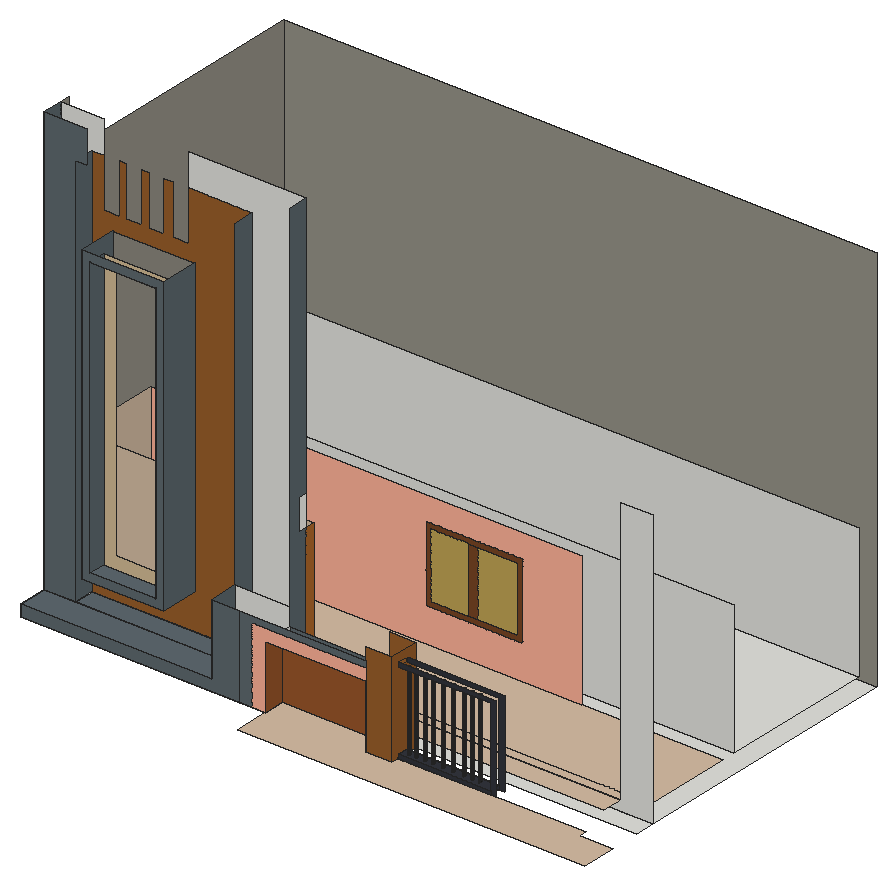
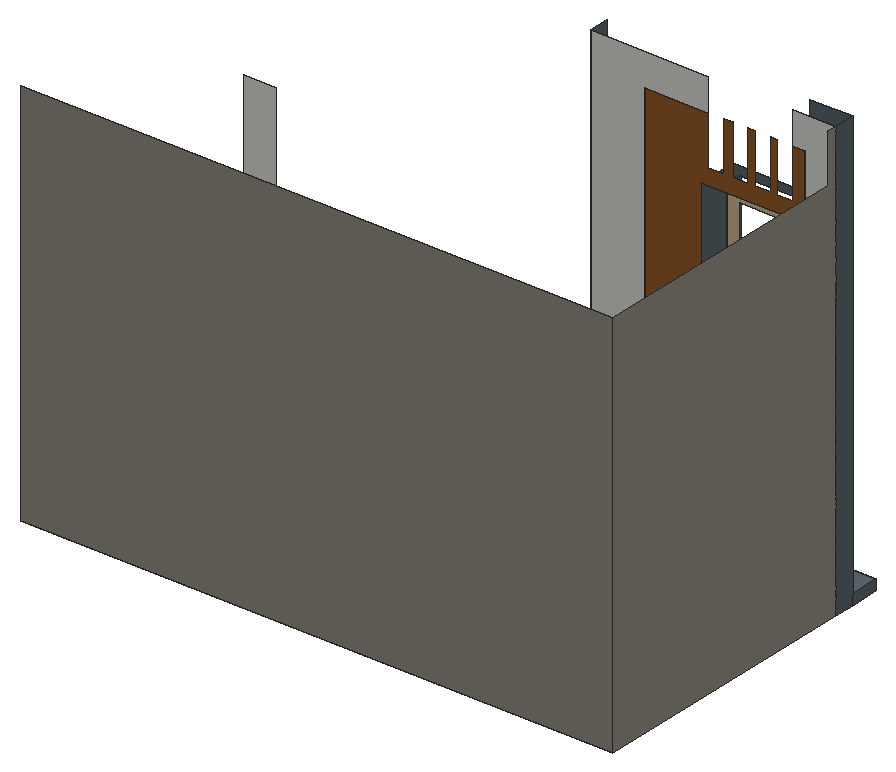
# SketchUp Ruby script. Lengths in inches.
U = 1.inch
M = Sketchup.active_model
def pt(a) = Geom::Point3d.new(a.map { |v| v * U })
def face(e, loops, mat)
  f = e.add_face(loops[0].map { |a| pt(a) })
  loops[1..].each { |l| e.add_face(l.map { |a| pt(a) }).erase! }
  f.material = f.back_material = mat if mat
  f
end
# faces: each face lists its corners as indices into pts; further lists are holes
def faces(e, pts, list, mat = nil) = list.each { |f| face(e, (f[0].is_a?(Array) ? f : [f]).map { |l| l.map { |i| pts[i] } }, mat) }
# xy, xz, yz: faces in a plane at the given z, y or x. An outline is a flat list of corners, or four numbers for a rectangle; further outlines are holes
def ring(l) = l.size == 4 ? [[l[0], l[1]], [l[2], l[1]], [l[2], l[3]], [l[0], l[3]]] : l.each_slice(2).to_a
def flat(e, list, mat, &to3) = list.each { |f| face(e, (f[0].is_a?(Array) ? f : [f]).map { |l| ring(l).map { |u, v| to3.(u, v) } }, mat) }
def xy(e, z, list, mat = nil) = flat(e, list, mat) { |x, y| [x, y, z] }
def xz(e, y, list, mat = nil) = flat(e, list, mat) { |x, z| [x, y, z] }
def yz(e, x, list, mat = nil) = flat(e, list, mat) { |y, z| [x, y, z] }
def lines(e, pts, list) = list.each { |a, b| e.add_line(pt(pts[a]), pt(pts[b])) }
# prism: a flat outline (further loops are holes) pulled along v
def prism(e, loops, v, mat = nil)
  f = face(e, loops, mat); d = Geom::Vector3d.new(v.map { |x| x * U })
  f.pushpull(f.normal.samedirection?(d) ? d.length : -d.length)
end
def box(e, o, s, mat = nil) = prism(e, [[o, [o[0] + s[0], o[1], o[2]], [o[0] + s[0], o[1] + s[1], o[2]], [o[0], o[1] + s[1], o[2]]]], [0, 0, s[2]], mat)
def at(x, y, z, deg = 0) = Geom::Transformation.translation(pt([x, y, z])) * Geom::Transformation.rotation(ORIGIN, Z_AXIS, deg.degrees)
def axes(o, x, y, z) = Geom::Transformation.new([*x, 0, *y, 0, *z, 0, *pt(o).to_a, 1])
def part(name) = M.definitions.add(name)
# library, detail: a bought-in or finely detailed component or shape, given as its bounding box
def library(name, o, s) = part(name).tap { |d| box(d.entities, o, s) }
def detail(e, o, s) = box(e.add_group.entities, o, s)
def put(e, d, t, mat = nil) = e.add_instance(d, t).tap { |i| i.material = mat if mat }
def group(e, t, mat = nil) = e.add_group.tap { |g| g.transformation = t; g.material = mat if mat }.entities
root = M.entities
M.materials.add("[Blinds Cloth Horizontal]").color = [192, 163, 85]
M.materials.add("[Color B02]").color = [255, 178, 153]
M.materials.add("[Color M08]").color = [30, 30, 30]
M.materials.add("[Formica Beige]").color = [211, 187, 149]
M.materials.add("[Formica Graystone]").color = [149, 146, 135]
M.materials.add("[Formica Laminate Dark]").color = [50, 53, 60]
M.materials.add("[Formica Laminate Light]").color = [213, 189, 164]
M.materials.add("[Formica Speckled Grey]").color = [94, 105, 111]
M.materials.add("[Wood Bamboo]").color = [177, 105, 43]
M.materials.add("[Wood Cherry Original]").color = [152, 86, 42]
M.materials.add("[Wood Floor Dark]").color = [153, 94, 42]
M.materials.add("[Wood Veneer 01]").color = [120, 70, 37]
xy(root,0,[[0,31.06,221.09,57.99],[311.65,31.06,335.09,57.99],[335.09,37.79,418.54,47.28],[221.09,49.81,311.65,57.99],[0,57.99,28.26,76.74],
  [28.26,57.99,172.2,76.74],[172.2,57.99,533.83,76.74],[0,76.74,533.83,328.17]])
xy(root,0,[[221.09,0,221.09,49.81,311.65,49.81,311.65,31.06,335.09,31.06,335.09,37.79,504.33,37.79,504.33,31.06,533.83,31.06,533.83,0]],"[Formica Laminate Light]")
xy(root,3.5625,[[[335.09,37.79,418.54,47.28],[412.31,41.58,412.05,41.61,411.81,41.71,411.6,41.875,411.44,42.08,411.34,42.32,411.31,42.58,411.34,42.84,411.44,43.08,411.6,43.29,411.81,43.45,412.05,43.55,412.31,43.58,412.57,43.55,412.81,43.45,413.02,43.29,413.18,43.08,413.27,42.84,413.31,42.58,413.27,42.32,413.18,42.08,413.02,41.875,412.81,41.71,412.57,41.61],[405.56,41.58,405.3,41.61,405.06,41.71,404.85,41.875,404.69,42.08,404.59,42.32,404.56,42.58,404.59,42.84,404.69,43.08,404.85,43.29,405.06,43.45,405.3,43.55,405.56,43.58,405.82,43.55,406.06,43.45,406.27,43.29,406.43,43.08,406.52,42.84,406.56,42.58,406.52,42.32,406.43,42.08,406.27,41.875,406.06,41.71,405.82,41.61],[398.25,41.58,397.99,41.61,397.75,41.71,397.54,41.875,397.38,42.08,397.28,42.32,397.25,42.58,397.28,42.84,397.38,43.08,397.54,43.29,397.75,43.45,397.99,43.55,398.25,43.58,398.51,43.55,398.75,43.45,398.95,43.29,399.11,43.08,399.21,42.84,399.25,42.58,399.21,42.32,399.11,42.08,398.95,41.875,398.75,41.71,398.51,41.61],[390.81,41.58,390.55,41.61,390.31,41.71,390.1,41.875,389.94,42.08,389.84,42.32,389.81,42.58,389.84,42.84,389.94,43.08,390.1,43.29,390.31,43.45,390.55,43.55,390.81,43.58,391.07,43.55,391.31,43.45,391.52,43.29,391.68,43.08,391.77,42.84,391.81,42.58,391.77,42.32,391.68,42.08,391.52,41.875,391.31,41.71,391.07,41.61],[381.12,41.58,380.86,41.61,380.62,41.71,380.41,41.875,380.26,42.08,380.16,42.32,380.12,42.58,380.16,42.84,380.26,43.08,380.41,43.29,380.62,43.45,380.86,43.55,381.12,43.58,381.38,43.55,381.62,43.45,381.83,43.29,381.99,43.08,382.09,42.84,382.12,42.58,382.09,42.32,381.99,42.08,381.83,41.875,381.62,41.71,381.38,41.61],[371.93,41.58,371.68,41.61,371.43,41.71,371.23,41.875,371.07,42.08,370.97,42.32,370.93,42.58,370.97,42.84,371.07,43.08,371.23,43.29,371.43,43.45,371.68,43.55,371.93,43.58,372.19,43.55,372.43,43.45,372.64,43.29,372.8,43.08,372.9,42.84,372.93,42.58,372.9,42.32,372.8,42.08,372.64,41.875,372.43,41.71,372.19,41.61],[363,41.58,362.74,41.61,362.5,41.71,362.29,41.875,362.13,42.08,362.03,42.32,362,42.58,362.03,42.84,362.13,43.08,362.29,43.29,362.5,43.45,362.74,43.55,363,43.58,363.26,43.55,363.5,43.45,363.7,43.29,363.86,43.08,363.96,42.84,364,42.58,363.96,42.32,363.86,42.08,363.7,41.875,363.5,41.71,363.26,41.61],[355.87,41.58,355.61,41.61,355.37,41.71,355.16,41.875,355.01,42.08,354.91,42.32,354.87,42.58,354.91,42.84,355.01,43.08,355.16,43.29,355.37,43.45,355.61,43.55,355.87,43.58,356.13,43.55,356.37,43.45,356.58,43.29,356.74,43.08,356.84,42.84,356.87,42.58,356.84,42.32,356.74,42.08,356.58,41.875,356.37,41.71,356.13,41.61],[348,41.58,347.74,41.61,347.5,41.71,347.29,41.875,347.13,42.08,347.03,42.32,347,42.58,347.03,42.84,347.13,43.08,347.29,43.29,347.5,43.45,347.74,43.55,348,43.58,348.26,43.55,348.5,43.45,348.7,43.29,348.86,43.08,348.96,42.84,349,42.58,348.96,42.32,348.86,42.08,348.7,41.875,348.5,41.71,348.26,41.61],[341.18,41.58,340.93,41.61,340.68,41.71,340.48,41.875,340.32,42.08,340.22,42.32,340.18,42.58,340.22,42.84,340.32,43.08,340.48,43.29,340.68,43.45,340.93,43.55,341.18,43.58,341.44,43.55,341.68,43.45,341.89,43.29,342.05,43.08,342.15,42.84,342.18,42.58,342.15,42.32,342.05,42.08,341.89,41.875,341.68,41.71,341.44,41.61]]],"[Formica Laminate Dark]")
xy(root,9,[[9,178.72,524.83,319.17]])
xy(root,9,[[221.09,57.99,504.33,76.74],[221.09,76.74,504.33,85.74],[9,85.74,524.83,166.38]],"[Formica Laminate Light]")
xy(root,9.8125,[[0,31.06,172.2,57.99],[28.26,57.99,172.2,76.74]],"[Formica Speckled Grey]")
xy(root,41.875,[[47,41.68,120.93,76.74]],"[Formica Speckled Grey]")
xy(root,49.15,[[54.27,41.68,113.66,56.99]],"[Formica Speckled Grey]")
xz(root,31.06,[[208.87,0,221.09,0,221.09,57.0625,311.65,57.0625,311.65,68.21,208.87,68.21]],"[Color B02]")
xz(root,31.06,[[0,0,196.64,0,196.64,73.875,172.2,73.875,172.2,9.8125,0,9.8125],[196.64,0,208.87,0,208.87,68.21,311.65,68.21,311.65,73.875,196.64,73.875]],"[Formica Speckled Grey]")
xz(root,31.06,[[311.65,0,335.09,84.875]],"[Wood Floor Dark]")
xz(root,37.79,[[335.09,0,418.54,3.5625],[418.54,0,423.6,0,423.6,77.6875,335.09,77.6875,335.09,74.1,418.54,74.1]],"[Formica Laminate Dark]")
xz(root,41.68,[[[47,41.875,120.93,307.5625],[54.27,49.15,113.66,300.29]]],"[Formica Speckled Grey]")
xz(root,47.28,[[335.09,0,418.54,3.5625],[418.54,0,418.54,74.1,335.09,74.1,335.09,77.6875,423.6,77.6875,423.6,0]],"[Formica Laminate Dark]")
xz(root,49.81,[[221.09,0,311.65,57.0625]],"[Wood Cherry Original]")
xz(root,56.99,[[[54.27,49.15,113.66,300.29],[65.18,60.06,102.75,289.38]]],"[Formica Beige]")
xz(root,57.99,[[0,0,28.26,9.8125],[28.26,0,172.2,9.8125],[172.2,0,221.09,73.875],[221.09,0,311.65,9],[311.65,0,335.09,9]])
xz(root,57.99,[[221.09,9,311.65,57.0625],[0,9.8125,28.26,9.8125,28.26,365.9375,38.68,365.9375,38.68,395.1875,0,395.1875]],"[Formica Speckled Grey]")
xz(root,57.99,[[311.65,9,335.09,84.875]],"[Wood Floor Dark]")
xz(root,76.74,[[0,0,0,395.1875,38.68,395.1875,38.68,365.9375,28.26,365.9375,28.26,0],[28.26,0,172.2,9.8125],[172.2,0,172.2,365.9375,115.05,365.9375,115.05,395.1875,221.09,395.1875,221.09,9,504.33,9,504.33,249,533.83,249,533.83,0]])
xz(root,76.74,[[[28.26,9.8125,172.2,9.8125,172.2,365.9375,115.05,365.9375,115.05,321.4375,100.98,321.4375,100.98,365.9375,93.18,365.9375,93.18,321.4375,79.11,321.4375,79.11,365.9375,72.8,365.9375,72.8,321.4375,58.74,321.4375,58.74,365.9375,52.74,365.9375,52.74,321.4375,38.68,321.4375,38.68,365.9375,28.26,365.9375],[47,41.875,120.93,307.5625]]],"[Wood Floor Dark]")
xz(root,85.74,[[9,9,221.09,129]],"[Formica Laminate Light]")
xz(root,166.38,[[261.47,44.26,294.83,103.46],[303.89,44.26,339.92,103.46]],"[Blinds Cloth Horizontal]")
xz(root,166.38,[[[9,9,398.15,129],[256.82,39.61,344.57,108.11]]],"[Color B02]")
xz(root,166.38,[[[256.82,39.61,344.57,108.11],[261.47,44.26,339.92,103.46]],[294.83,44.26,303.89,103.46]],"[Wood Veneer 01]")
xz(root,178.72,[[9,9,524.83,129]])
xz(root,319.17,[[9,9,524.83,129]])
xz(root,328.17,[[0,0,533.83,350.875]],"[Formica Graystone]")
yz(root,0,[[76.74,0,76.74,395.1875,85.74,395.1875,85.74,350.875,328.17,350.875,328.17,0]],"[Formica Graystone]")
yz(root,0,[[31.06,0,57.99,9.8125],[57.99,0,76.74,395.1875]],"[Formica Speckled Grey]")
yz(root,9,[[178.72,9,319.17,129]])
yz(root,9,[[85.74,9,166.38,129]],"[Formica Laminate Light]")
yz(root,28.26,[[57.99,0,76.74,9.8125]])
yz(root,28.26,[[57.99,9.8125,76.74,365.9375]],"[Formica Speckled Grey]")
yz(root,47,[[41.68,41.875,76.74,307.5625]],"[Formica Speckled Grey]")
yz(root,54.27,[[41.68,49.15,56.99,300.29]],"[Formica Speckled Grey]")
yz(root,113.66,[[41.68,49.15,56.99,300.29]],"[Formica Speckled Grey]")
yz(root,120.93,[[41.68,41.875,76.74,307.5625]],"[Formica Speckled Grey]")
yz(root,172.2,[[57.99,0,76.74,9.8125]])
yz(root,172.2,[[31.06,9.8125,57.99,73.875],[57.99,9.8125,76.74,365.9375]],"[Formica Speckled Grey]")
yz(root,221.09,[[49.81,0,57.99,57.0625]])
yz(root,221.09,[[57.99,9,76.74,9,76.74,129,68.99,129,68.99,157,76.74,157,76.74,395.1875,57.99,395.1875]],"[Formica Speckled Grey]")
yz(root,221.09,[[76.74,9,85.74,129]],"[Wood Bamboo]")
yz(root,221.09,[[31.06,0,49.81,57.0625]],"[Wood Cherry Original]")
yz(root,311.65,[[31.06,0,49.81,57.0625]],"[Wood Cherry Original]")
yz(root,335.09,[[37.79,0,47.28,3.5625]])
yz(root,335.09,[[[31.06,0,37.79,0,37.79,3.5625,47.28,3.5625,47.28,0,57.99,0,57.99,84.875,31.06,84.875],[37.79,74.1,47.28,77.6875]]],"[Wood Floor Dark]")
p = [[340.93,41.61,74.1],[340.68,41.71,74.1],[340.68,41.71,3.5625],[340.93,41.61,3.5625],[341.18,41.58,74.1],[341.18,41.58,3.5625],
  [341.44,41.61,74.1],[341.44,41.61,3.5625],[341.68,41.71,74.1],[341.68,41.71,3.5625],[347.74,41.61,74.1],[347.5,41.71,74.1],
  [347.5,41.71,3.5625],[347.74,41.61,3.5625],[348,41.58,74.1],[348,41.58,3.5625],[348.26,41.61,74.1],[348.26,41.61,3.5625],
  [348.5,41.71,74.1],[348.5,41.71,3.5625],[355.61,41.61,74.1],[355.37,41.71,74.1],[355.37,41.71,3.5625],[355.61,41.61,3.5625],
  [355.87,41.58,74.1],[355.87,41.58,3.5625],[356.13,41.61,74.1],[356.13,41.61,3.5625],[356.37,41.71,74.1],[356.37,41.71,3.5625],
  [362.74,41.61,74.1],[362.5,41.71,74.1],[362.5,41.71,3.5625],[362.74,41.61,3.5625],[363,41.58,74.1],[363,41.58,3.5625],
  [363.26,41.61,74.1],[363.26,41.61,3.5625],[363.5,41.71,74.1],[363.5,41.71,3.5625],[371.68,41.61,74.1],[371.43,41.71,74.1],
  [371.43,41.71,3.5625],[371.68,41.61,3.5625],[371.93,41.58,74.1],[371.93,41.58,3.5625],[372.19,41.61,74.1],[372.19,41.61,3.5625],
  [372.43,41.71,74.1],[372.43,41.71,3.5625],[380.86,41.61,74.1],[380.62,41.71,74.1],[380.62,41.71,3.5625],[380.86,41.61,3.5625],
  [381.12,41.58,74.1],[381.12,41.58,3.5625],[381.38,41.61,74.1],[381.38,41.61,3.5625],[381.62,41.71,74.1],[381.62,41.71,3.5625],
  [390.55,41.61,74.1],[390.31,41.71,74.1],[390.31,41.71,3.5625],[390.55,41.61,3.5625],[390.81,41.58,74.1],[390.81,41.58,3.5625],
  [391.07,41.61,74.1],[391.07,41.61,3.5625],[391.31,41.71,74.1],[391.31,41.71,3.5625],[397.99,41.61,74.1],[397.75,41.71,74.1],
  [397.75,41.71,3.5625],[397.99,41.61,3.5625],[398.25,41.58,74.1],[398.25,41.58,3.5625],[398.51,41.61,74.1],[398.51,41.61,3.5625],
  [398.75,41.71,74.1],[398.75,41.71,3.5625],[405.3,41.61,74.1],[405.06,41.71,74.1],[405.06,41.71,3.5625],[405.3,41.61,3.5625],
  [405.56,41.58,74.1],[405.56,41.58,3.5625],[405.82,41.61,74.1],[405.82,41.61,3.5625],[406.06,41.71,74.1],[406.06,41.71,3.5625],
  [340.48,41.875,74.1],[340.48,41.875,3.5625],[341.89,41.875,74.1],[341.89,41.875,3.5625],[347.29,41.875,74.1],[347.29,41.875,3.5625],
  [348.7,41.875,74.1],[348.7,41.875,3.5625],[355.16,41.875,74.1],[355.16,41.875,3.5625],[356.58,41.875,74.1],[356.58,41.875,3.5625],
  [362.29,41.875,74.1],[362.29,41.875,3.5625],[363.7,41.875,74.1],[363.7,41.875,3.5625],[371.23,41.875,74.1],[371.23,41.875,3.5625],
  [372.64,41.875,74.1],[372.64,41.875,3.5625],[380.41,41.875,74.1],[380.41,41.875,3.5625],[381.83,41.875,74.1],[381.83,41.875,3.5625],
  [390.1,41.875,74.1],[390.1,41.875,3.5625],[391.52,41.875,74.1],[391.52,41.875,3.5625],[397.54,41.875,74.1],[397.54,41.875,3.5625],
  [398.95,41.875,74.1],[398.95,41.875,3.5625],[404.85,41.875,74.1],[404.85,41.875,3.5625],[340.32,42.08,74.1],[340.32,42.08,3.5625],
  [342.05,42.08,74.1],[342.05,42.08,3.5625],[347.13,42.08,74.1],[347.13,42.08,3.5625],[348.86,42.08,74.1],[348.86,42.08,3.5625],
  [355.01,42.08,74.1],[355.01,42.08,3.5625],[356.74,42.08,74.1],[356.74,42.08,3.5625],[362.13,42.08,74.1],[362.13,42.08,3.5625],
  [363.86,42.08,74.1],[363.86,42.08,3.5625],[371.07,42.08,74.1],[371.07,42.08,3.5625],[372.8,42.08,74.1],[372.8,42.08,3.5625],
  [380.26,42.08,74.1],[380.26,42.08,3.5625],[381.99,42.08,74.1],[381.99,42.08,3.5625],[389.94,42.08,74.1],[389.94,42.08,3.5625],
  [391.68,42.08,74.1],[391.68,42.08,3.5625],[397.38,42.08,74.1],[397.38,42.08,3.5625],[399.11,42.08,74.1],[399.11,42.08,3.5625],
  [404.69,42.08,74.1],[404.69,42.08,3.5625],[340.22,42.32,74.1],[340.22,42.32,3.5625],[342.15,42.32,74.1],[342.15,42.32,3.5625],
  [347.03,42.32,74.1],[347.03,42.32,3.5625],[348.96,42.32,74.1],[348.96,42.32,3.5625],[354.91,42.32,74.1],[354.91,42.32,3.5625],
  [356.84,42.32,74.1],[356.84,42.32,3.5625],[362.03,42.32,74.1],[362.03,42.32,3.5625],[363.96,42.32,74.1],[363.96,42.32,3.5625],
  [370.97,42.32,74.1],[370.97,42.32,3.5625],[372.9,42.32,74.1],[372.9,42.32,3.5625],[380.16,42.32,74.1],[380.16,42.32,3.5625],
  [382.09,42.32,74.1],[382.09,42.32,3.5625],[389.84,42.32,74.1],[389.84,42.32,3.5625],[391.77,42.32,74.1],[391.77,42.32,3.5625],
  [397.28,42.32,74.1],[397.28,42.32,3.5625],[399.21,42.32,74.1],[399.21,42.32,3.5625],[404.59,42.32,74.1],[404.59,42.32,3.5625],
  [340.18,42.58,74.1],[340.18,42.58,3.5625],[342.18,42.58,74.1],[342.18,42.58,3.5625],[347,42.58,74.1],[347,42.58,3.5625],
  [349,42.58,74.1],[349,42.58,3.5625],[354.87,42.58,74.1],[354.87,42.58,3.5625],[356.87,42.58,74.1],[356.87,42.58,3.5625],
  [362,42.58,74.1],[362,42.58,3.5625],[364,42.58,74.1],[364,42.58,3.5625],[370.93,42.58,74.1],[370.93,42.58,3.5625],
  [372.93,42.58,74.1],[372.93,42.58,3.5625],[380.12,42.58,74.1],[380.12,42.58,3.5625],[382.12,42.58,74.1],[382.12,42.58,3.5625],
  [389.81,42.58,74.1],[389.81,42.58,3.5625],[391.81,42.58,74.1],[391.81,42.58,3.5625],[397.25,42.58,74.1],[397.25,42.58,3.5625],
  [399.25,42.58,74.1],[399.25,42.58,3.5625],[404.56,42.58,74.1],[404.56,42.58,3.5625],[340.22,42.84,74.1],[340.22,42.84,3.5625],
  [342.15,42.84,74.1],[342.15,42.84,3.5625],[347.03,42.84,74.1],[347.03,42.84,3.5625],[348.96,42.84,74.1],[348.96,42.84,3.5625],
  [354.91,42.84,74.1],[354.91,42.84,3.5625],[356.84,42.84,74.1],[356.84,42.84,3.5625],[362.03,42.84,74.1],[362.03,42.84,3.5625],
  [363.96,42.84,74.1],[363.96,42.84,3.5625],[370.97,42.84,74.1],[370.97,42.84,3.5625],[372.9,42.84,74.1],[372.9,42.84,3.5625],
  [380.16,42.84,74.1],[380.16,42.84,3.5625],[382.09,42.84,74.1],[382.09,42.84,3.5625],[389.84,42.84,74.1],[389.84,42.84,3.5625],
  [391.77,42.84,74.1],[391.77,42.84,3.5625],[397.28,42.84,74.1],[397.28,42.84,3.5625],[399.21,42.84,74.1],[399.21,42.84,3.5625],
  [404.59,42.84,74.1],[404.59,42.84,3.5625],[340.32,43.08,74.1],[340.32,43.08,3.5625],[342.05,43.08,74.1],[342.05,43.08,3.5625],
  [347.13,43.08,74.1],[347.13,43.08,3.5625],[348.86,43.08,74.1],[348.86,43.08,3.5625],[355.01,43.08,74.1],[355.01,43.08,3.5625],
  [356.74,43.08,74.1],[356.74,43.08,3.5625],[362.13,43.08,74.1],[362.13,43.08,3.5625],[363.86,43.08,74.1],[363.86,43.08,3.5625],
  [371.07,43.08,74.1],[371.07,43.08,3.5625],[372.8,43.08,74.1],[372.8,43.08,3.5625],[380.26,43.08,74.1],[380.26,43.08,3.5625],
  [381.99,43.08,74.1],[381.99,43.08,3.5625],[389.94,43.08,74.1],[389.94,43.08,3.5625],[391.68,43.08,74.1],[391.68,43.08,3.5625],
  [397.38,43.08,74.1],[397.38,43.08,3.5625],[399.11,43.08,74.1],[399.11,43.08,3.5625],[404.69,43.08,74.1],[404.69,43.08,3.5625],
  [340.48,43.29,74.1],[340.48,43.29,3.5625],[341.89,43.29,74.1],[341.89,43.29,3.5625],[347.29,43.29,74.1],[347.29,43.29,3.5625],
  [348.7,43.29,74.1],[348.7,43.29,3.5625],[355.16,43.29,74.1],[355.16,43.29,3.5625],[356.58,43.29,74.1],[356.58,43.29,3.5625],
  [362.29,43.29,74.1],[362.29,43.29,3.5625],[363.7,43.29,74.1],[363.7,43.29,3.5625],[371.23,43.29,74.1],[371.23,43.29,3.5625],
  [372.64,43.29,74.1],[372.64,43.29,3.5625],[380.41,43.29,74.1],[380.41,43.29,3.5625],[381.83,43.29,74.1],[381.83,43.29,3.5625],
  [390.1,43.29,74.1],[390.1,43.29,3.5625],[391.52,43.29,74.1],[391.52,43.29,3.5625],[397.54,43.29,74.1],[397.54,43.29,3.5625],
  [398.95,43.29,74.1],[398.95,43.29,3.5625],[404.85,43.29,74.1],[404.85,43.29,3.5625],[340.68,43.45,74.1],[340.68,43.45,3.5625],
  [341.68,43.45,74.1],[341.68,43.45,3.5625],[347.5,43.45,74.1],[347.5,43.45,3.5625],[348.5,43.45,74.1],[348.5,43.45,3.5625],
  [355.37,43.45,74.1],[355.37,43.45,3.5625],[356.37,43.45,74.1],[356.37,43.45,3.5625],[362.5,43.45,74.1],[362.5,43.45,3.5625],
  [363.5,43.45,74.1],[363.5,43.45,3.5625],[371.43,43.45,74.1],[371.43,43.45,3.5625],[372.43,43.45,74.1],[372.43,43.45,3.5625],
  [380.62,43.45,74.1],[380.62,43.45,3.5625],[381.62,43.45,74.1],[381.62,43.45,3.5625],[390.31,43.45,74.1],[390.31,43.45,3.5625],
  [391.31,43.45,74.1],[391.31,43.45,3.5625],[397.75,43.45,74.1],[397.75,43.45,3.5625],[398.75,43.45,74.1],[398.75,43.45,3.5625],
  [405.06,43.45,74.1],[405.06,43.45,3.5625],[340.93,43.55,74.1],[340.93,43.55,3.5625],[341.44,43.55,74.1],[341.44,43.55,3.5625],
  [347.74,43.55,74.1],[347.74,43.55,3.5625],[348.26,43.55,74.1],[348.26,43.55,3.5625],[355.61,43.55,74.1],[355.61,43.55,3.5625],
  [356.13,43.55,74.1],[356.13,43.55,3.5625],[362.74,43.55,74.1],[362.74,43.55,3.5625],[363.26,43.55,74.1],[363.26,43.55,3.5625],
  [371.68,43.55,74.1],[371.68,43.55,3.5625],[372.19,43.55,74.1],[372.19,43.55,3.5625],[380.86,43.55,74.1],[380.86,43.55,3.5625],
  [381.38,43.55,74.1],[381.38,43.55,3.5625],[390.55,43.55,74.1],[390.55,43.55,3.5625],[391.07,43.55,74.1],[391.07,43.55,3.5625],
  [397.99,43.55,74.1],[397.99,43.55,3.5625],[398.51,43.55,74.1],[398.51,43.55,3.5625],[405.3,43.55,74.1],[405.3,43.55,3.5625],
  [341.18,43.58,74.1],[341.18,43.58,3.5625],[348,43.58,74.1],[348,43.58,3.5625],[355.87,43.58,74.1],[355.87,43.58,3.5625],
  [363,43.58,74.1],[363,43.58,3.5625],[371.93,43.58,74.1],[371.93,43.58,3.5625],[381.12,43.58,74.1],[381.12,43.58,3.5625],
  [390.81,43.58,74.1],[390.81,43.58,3.5625],[398.25,43.58,74.1],[398.25,43.58,3.5625],[405.56,43.58,74.1],[405.56,43.58,3.5625],
  [405.82,43.55,74.1],[405.82,43.55,3.5625]]
faces(root,p,[[0,1,2,3],[4,0,3,5],[6,4,5,7],[8,6,7,9],[10,11,12,13],[14,10,13,15],[16,14,15,17],[18,16,17,19],
  [20,21,22,23],[24,20,23,25],[26,24,25,27],[28,26,27,29],[30,31,32,33],[34,30,33,35],[36,34,35,37],[38,36,37,39],
  [40,41,42,43],[44,40,43,45],[46,44,45,47],[48,46,47,49],[50,51,52,53],[54,50,53,55],[56,54,55,57],[58,56,57,59],
  [60,61,62,63],[64,60,63,65],[66,64,65,67],[68,66,67,69],[70,71,72,73],[74,70,73,75],[76,74,75,77],[78,76,77,79],
  [80,81,82,83],[84,80,83,85],[86,84,85,87],[88,86,87,89],[1,90,91,2],[92,8,9,93],[11,94,95,12],[96,18,19,97],
  [21,98,99,22],[100,28,29,101],[31,102,103,32],[104,38,39,105],[41,106,107,42],[108,48,49,109],[51,110,111,52],[112,58,59,113],
  [61,114,115,62],[116,68,69,117],[71,118,119,72],[120,78,79,121],[81,122,123,82],[90,124,125,91],[126,92,93,127],[94,128,129,95],
  [130,96,97,131],[98,132,133,99],[134,100,101,135],[102,136,137,103],[138,104,105,139],[106,140,141,107],[142,108,109,143],[110,144,145,111],
  [146,112,113,147],[114,148,149,115],[150,116,117,151],[118,152,153,119],[154,120,121,155],[122,156,157,123],[124,158,159,125],[160,126,127,161],
  [128,162,163,129],[164,130,131,165],[132,166,167,133],[168,134,135,169],[136,170,171,137],[172,138,139,173],[140,174,175,141],[176,142,143,177],
  [144,178,179,145],[180,146,147,181],[148,182,183,149],[184,150,151,185],[152,186,187,153],[188,154,155,189],[156,190,191,157],[158,192,193,159],
  [194,160,161,195],[162,196,197,163],[198,164,165,199],[166,200,201,167],[202,168,169,203],[170,204,205,171],[206,172,173,207],[174,208,209,175],
  [210,176,177,211],[178,212,213,179],[214,180,181,215],[182,216,217,183],[218,184,185,219],[186,220,221,187],[222,188,189,223],[190,224,225,191],
  [192,226,227,193],[228,194,195,229],[196,230,231,197],[232,198,199,233],[200,234,235,201],[236,202,203,237],[204,238,239,205],[240,206,207,241],
  [208,242,243,209],[244,210,211,245],[212,246,247,213],[248,214,215,249],[216,250,251,217],[252,218,219,253],[220,254,255,221],[256,222,223,257],
  [224,258,259,225],[226,260,261,227],[262,228,229,263],[230,264,265,231],[266,232,233,267],[234,268,269,235],[270,236,237,271],[238,272,273,239],
  [274,240,241,275],[242,276,277,243],[278,244,245,279],[246,280,281,247],[282,248,249,283],[250,284,285,251],[286,252,253,287],[254,288,289,255],
  [290,256,257,291],[258,292,293,259],[260,294,295,261],[296,262,263,297],[264,298,299,265],[300,266,267,301],[268,302,303,269],[304,270,271,305],
  [272,306,307,273],[308,274,275,309],[276,310,311,277],[312,278,279,313],[280,314,315,281],[316,282,283,317],[284,318,319,285],[320,286,287,321],
  [288,322,323,289],[324,290,291,325],[292,326,327,293],[294,328,329,295],[330,296,297,331],[298,332,333,299],[334,300,301,335],[302,336,337,303],
  [338,304,305,339],[306,340,341,307],[342,308,309,343],[310,344,345,311],[346,312,313,347],[314,348,349,315],[350,316,317,351],[318,352,353,319],
  [354,320,321,355],[322,356,357,323],[358,324,325,359],[326,360,361,327],[328,362,363,329],[364,330,331,365],[332,366,367,333],[368,334,335,369],
  [336,370,371,337],[372,338,339,373],[340,374,375,341],[376,342,343,377],[344,378,379,345],[380,346,347,381],[348,382,383,349],[384,350,351,385],
  [352,386,387,353],[388,354,355,389],[356,390,391,357],[392,358,359,393],[360,394,395,361],[362,396,397,363],[396,364,365,397],[366,398,399,367],
  [398,368,369,399],[370,400,401,371],[400,372,373,401],[374,402,403,375],[402,376,377,403],[378,404,405,379],[404,380,381,405],[382,406,407,383],
  [406,384,385,407],[386,408,409,387],[408,388,389,409],[390,410,411,391],[410,392,393,411],[394,412,413,395],[412,414,415,413]],"[Color M08]")
